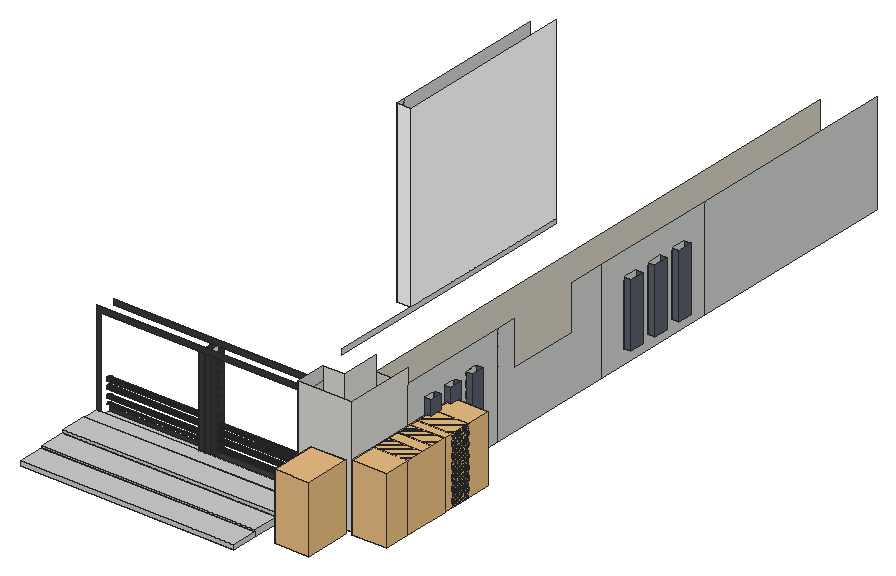
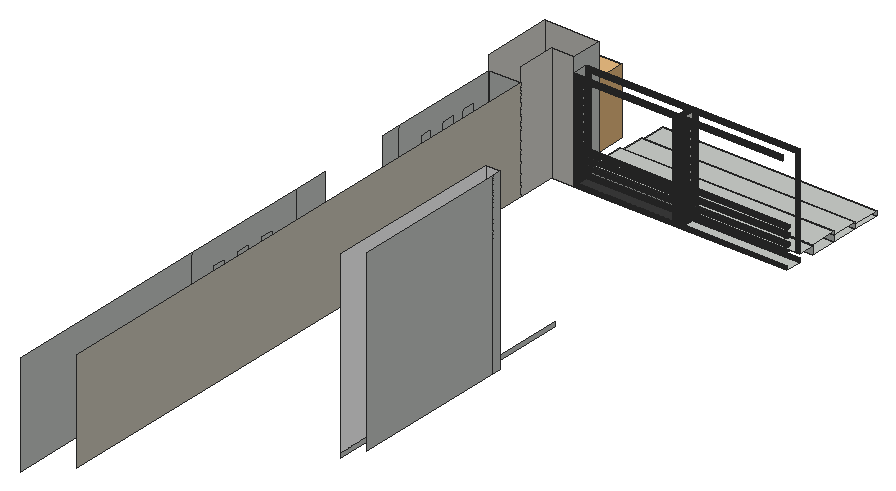
# SketchUp Ruby script. Lengths in inches.
U = 1.inch
M = Sketchup.active_model
def pt(a) = Geom::Point3d.new(a.map { |v| v * U })
def face(e, loops, mat)
  f = e.add_face(loops[0].map { |a| pt(a) })
  loops[1..].each { |l| e.add_face(l.map { |a| pt(a) }).erase! }
  f.material = f.back_material = mat if mat
  f
end
# faces: each face lists its corners as indices into pts; further lists are holes
def faces(e, pts, list, mat = nil) = list.each { |f| face(e, (f[0].is_a?(Array) ? f : [f]).map { |l| l.map { |i| pts[i] } }, mat) }
# xy, xz, yz: faces in a plane at the given z, y or x. An outline is a flat list of corners, or four numbers for a rectangle; further outlines are holes
def ring(l) = l.size == 4 ? [[l[0], l[1]], [l[2], l[1]], [l[2], l[3]], [l[0], l[3]]] : l.each_slice(2).to_a
def flat(e, list, mat, &to3) = list.each { |f| face(e, (f[0].is_a?(Array) ? f : [f]).map { |l| ring(l).map { |u, v| to3.(u, v) } }, mat) }
def xy(e, z, list, mat = nil) = flat(e, list, mat) { |x, y| [x, y, z] }
def xz(e, y, list, mat = nil) = flat(e, list, mat) { |x, z| [x, y, z] }
def yz(e, x, list, mat = nil) = flat(e, list, mat) { |y, z| [x, y, z] }
def lines(e, pts, list) = list.each { |a, b| e.add_line(pt(pts[a]), pt(pts[b])) }
# prism: a flat outline (further loops are holes) pulled along v
def prism(e, loops, v, mat = nil)
  f = face(e, loops, mat); d = Geom::Vector3d.new(v.map { |x| x * U })
  f.pushpull(f.normal.samedirection?(d) ? d.length : -d.length)
end
def box(e, o, s, mat = nil) = prism(e, [[o, [o[0] + s[0], o[1], o[2]], [o[0] + s[0], o[1] + s[1], o[2]], [o[0], o[1] + s[1], o[2]]]], [0, 0, s[2]], mat)
def at(x, y, z, deg = 0) = Geom::Transformation.translation(pt([x, y, z])) * Geom::Transformation.rotation(ORIGIN, Z_AXIS, deg.degrees)
def axes(o, x, y, z) = Geom::Transformation.new([*x, 0, *y, 0, *z, 0, *pt(o).to_a, 1])
def part(name) = M.definitions.add(name)
# library, detail: a bought-in or finely detailed component or shape, given as its bounding box
def library(name, o, s) = part(name).tap { |d| box(d.entities, o, s) }
def detail(e, o, s) = box(e.add_group.entities, o, s)
def put(e, d, t, mat = nil) = e.add_instance(d, t).tap { |i| i.material = mat if mat }
def group(e, t, mat = nil) = e.add_group.tap { |g| g.transformation = t; g.material = mat if mat }.entities
root = M.entities
M.materials.add("[Basic Tile]").color = [203, 206, 202]
M.materials.add("[Color M00]").color = [255, 255, 255]
M.materials.add("[Color M07]").color = [58, 58, 58]
M.materials.add("[Formica Graystone]").color = [209, 204, 189]
M.materials.add("[Formica Laminate Dark]").color = [89, 94, 107]
M.materials.add("[Terrazzo Tile Light]").color = [219, 217, 210]
c1 = library("chau cay",[-24.34,-109.24,0],[56.46,62.58,79.69])
xy(root,0,[[1126.47,137.11,1535.88,187.89],[1126.47,187.89,1535.88,238.67],[1126.47,238.67,1535.88,289.93],[1535.88,289.93,1535.88,350.55,1578.42,350.55,1578.42,424.2,1639.03,424.2,1639.03,289.93],[1126.47,320.24,1535.88,350.55]],"[Basic Tile]")
xy(root,8.3125,[[1322.28,320.24,1333.57,350.55]])
xy(root,8.3125,[[1527,320.24,1535.88,350.55]],"[Basic Tile]")
xy(root,8.3125,[[1344.86,320.24,1527,350.55]],"[Color M07]")
xy(root,8.4375,[[1126.47,137.11,1535.88,187.89]],"[Basic Tile]")
xy(root,11.8125,[[1126.47,187.89,1535.88,238.67]],"[Basic Tile]")
xy(root,15.5,[[1126.47,289.93,1535.88,320.24]],"[Basic Tile]")
xy(root,17.75,[[1126.47,238.67,1535.88,289.93]],"[Basic Tile]")
xy(root,27.29,[[1639.03,943.34,1652.28,971.59],[1639.03,1000.59,1652.28,1028.84],[1639.03,1058.41,1652.28,1086.66]],"[Formica Laminate Dark]")
xy(root,31.8125,[[1639.03,462.79,1652.28,487.66],[1639.03,510.85,1652.28,535.72],[1639.03,562.72,1652.28,587.6]],"[Formica Laminate Dark]")
xz(root,137.11,[[1126.47,0,1535.88,8.4375]],"[Basic Tile]")
xz(root,187.89,[[1126.47,0,1535.88,8.4375],[1126.47,8.4375,1535.88,11.8125]],"[Basic Tile]")
xz(root,238.67,[[1126.47,0,1535.88,11.8125],[1126.47,11.8125,1535.88,17.75]],"[Basic Tile]")
xz(root,289.93,[[1126.47,0,1535.88,15.5],[1126.47,15.5,1535.88,17.75]],"[Basic Tile]")
xz(root,289.93,[[1535.88,0,1639.03,222.4375]],"[Terrazzo Tile Light]")
xz(root,320.24,[[1344.86,8.3125,1527,15.5]],"[Basic Tile]")
xz(root,320.24,[[1126.47,0,1535.88,8.3125],[1322.28,8.3125,1333.57,15.5],[1333.57,8.3125,1344.86,15.5],[1527,8.3125,1535.88,15.5],[1126.47,15.5,1134.85,15.5,1134.85,184.74,1527,184.74,1527,15.5,1535.88,15.5,1535.88,195.17,1126.47,195.17],
  [1322.28,15.5,1333.57,184.74],[1333.57,15.5,1344.86,184.74]],"[Color M07]")
xz(root,350.55,[[1126.47,0,1126.47,8.3125,1333.57,8.3125,1333.57,184.74,1344.86,184.74,1344.86,8.3125,1535.88,8.3125,1535.88,0],[1527,8.3125,1527,184.74,1134.85,184.74,1134.85,195.17,1535.88,195.17,1535.88,8.3125],[1322.28,8.3125,1333.57,184.74]],"[Color M07]")
xz(root,350.55,[[1535.88,0,1578.42,222.4375]],"[Terrazzo Tile Light]")
xz(root,424.2,[[1578.42,0,1639.03,194.8125]],"[Basic Tile]")
xz(root,462.79,[[1639.03,31.8125,1652.28,155.0625]],"[Formica Laminate Dark]")
xz(root,487.66,[[1639.03,31.8125,1652.28,155.0625]],"[Formica Laminate Dark]")
xz(root,510.85,[[1639.03,31.8125,1652.28,155.0625]],"[Formica Laminate Dark]")
xz(root,535.72,[[1639.03,31.8125,1652.28,155.0625]],"[Formica Laminate Dark]")
xz(root,562.72,[[1639.03,31.8125,1652.28,155.0625]],"[Formica Laminate Dark]")
xz(root,587.6,[[1639.03,31.8125,1652.28,155.0625]],"[Formica Laminate Dark]")
xz(root,868.79,[[1262.85,9,1290.28,349.625]],"[Color M00]")
xz(root,943.34,[[1639.03,27.29,1652.28,149.91]],"[Formica Laminate Dark]")
xz(root,971.59,[[1639.03,27.29,1652.28,149.91]],"[Formica Laminate Dark]")
xz(root,1000.59,[[1639.03,27.29,1652.28,149.91]],"[Formica Laminate Dark]")
xz(root,1028.84,[[1639.03,27.29,1652.28,149.91]],"[Formica Laminate Dark]")
xz(root,1058.41,[[1639.03,27.29,1652.28,149.91]],"[Formica Laminate Dark]")
xz(root,1086.66,[[1639.03,27.29,1652.28,149.91]],"[Formica Laminate Dark]")
yz(root,1262.85,[[868.79,9,886.125,349.625],[886.125,9,1187.61,349.625]],"[Basic Tile]")
yz(root,1290.28,[[703.09,0,1215.04,9]],"[Basic Tile]")
yz(root,1290.28,[[868.79,9,1215.04,349.625]],"[Color M00]")
yz(root,1322.28,[[[320.24,8.3125,350.55,184.74],[337.34,16.89,338.33,17.02,339.25,17.4,340.04,18.01,340.64,18.8,341.02,19.72,341.15,20.71,341.02,21.69,340.64,22.61,340.04,23.4,339.25,24.01,338.33,24.39,337.34,24.52,336.35,24.39,335.43,24.01,334.65,23.4,334.04,22.61,333.66,21.69,333.53,20.71,333.66,19.72,334.04,18.8,334.65,18.01,335.43,17.4,336.35,17.02],[337.34,31.39,338.33,31.52,339.25,31.9,340.04,32.51,340.64,33.3,341.02,34.22,341.15,35.21,341.02,36.19,340.64,37.11,340.04,37.9,339.25,38.51,338.33,38.89,337.34,39.02,336.35,38.89,335.43,38.51,334.65,37.9,334.04,37.11,333.66,36.19,333.53,35.21,333.66,34.22,334.04,33.3,334.65,32.51,335.43,31.9,336.35,31.52],[337.34,47.21,338.33,47.34,339.25,47.72,340.04,48.32,340.64,49.11,341.02,50.03,341.15,51.02,341.02,52,340.64,52.92,340.04,53.71,339.25,54.32,338.33,54.7,337.34,54.83,336.35,54.7,335.43,54.32,334.65,53.71,334.04,52.92,333.66,52,333.53,51.02,333.66,50.03,334.04,49.11,334.65,48.32,335.43,47.72,336.35,47.34],[337.34,61.64,338.33,61.77,339.25,62.15,340.04,62.76,340.64,63.55,341.02,64.47,341.15,65.46,341.02,66.44,340.64,67.36,340.04,68.15,339.25,68.76,338.33,69.14,337.34,69.27,336.35,69.14,335.43,68.76,334.65,68.15,334.04,67.36,333.66,66.44,333.53,65.46,333.66,64.47,334.04,63.55,334.65,62.76,335.43,62.15,336.35,61.77],[337.34,76.33,338.33,76.46,339.25,76.84,340.04,77.45,340.64,78.24,341.02,79.16,341.15,80.14,341.02,81.13,340.64,82.05,340.04,82.84,339.25,83.44,338.33,83.83,337.34,83.96,336.35,83.83,335.43,83.44,334.65,82.84,334.04,82.05,333.66,81.13,333.53,80.14,333.66,79.16,334.04,78.24,334.65,77.45,335.43,76.84,336.35,76.46],[337.34,90.83,338.33,90.96,339.25,91.34,340.04,91.95,340.64,92.74,341.02,93.66,341.15,94.64,341.02,95.63,340.64,96.55,340.04,97.34,339.25,97.94,338.33,98.33,337.34,98.46,336.35,98.33,335.43,97.94,334.65,97.34,334.04,96.55,333.66,95.63,333.53,94.64,333.66,93.66,334.04,92.74,334.65,91.95,335.43,91.34,336.35,90.96],[337.34,103.39,338.33,103.52,339.25,103.9,340.04,104.51,340.64,105.3,341.02,106.22,341.15,107.21,341.02,108.19,340.64,109.11,340.04,109.9,339.25,110.51,338.33,110.89,337.34,111.02,336.35,110.89,335.43,110.51,334.65,109.9,334.04,109.11,333.66,108.19,333.53,107.21,333.66,106.22,334.04,105.3,334.65,104.51,335.43,103.9,336.35,103.52],[337.34,117.89,338.33,118.02,339.25,118.4,340.04,119.01,340.64,119.8,341.02,120.72,341.15,121.71,341.02,122.69,340.64,123.61,340.04,124.4,339.25,125.01,338.33,125.39,337.34,125.52,336.35,125.39,335.43,125.01,334.65,124.4,334.04,123.61,333.66,122.69,333.53,121.71,333.66,120.72,334.04,119.8,334.65,119.01,335.43,118.4,336.35,118.02],[337.34,134.02,338.33,134.15,339.25,134.53,340.04,135.13,340.64,135.92,341.02,136.84,341.15,137.83,341.02,138.82,340.64,139.74,340.04,140.53,339.25,141.13,338.33,141.51,337.34,141.64,336.35,141.51,335.43,141.13,334.65,140.53,334.04,139.74,333.66,138.82,333.53,137.83,333.66,136.84,334.04,135.92,334.65,135.13,335.43,134.53,336.35,134.15],[337.34,147.52,338.33,147.65,339.25,148.03,340.04,148.63,340.64,149.42,341.02,150.34,341.15,151.33,341.02,152.32,340.64,153.24,340.04,154.03,339.25,154.63,338.33,155.01,337.34,155.14,336.35,155.01,335.43,154.63,334.65,154.03,334.04,153.24,333.66,152.32,333.53,151.33,333.66,150.34,334.04,149.42,334.65,148.63,335.43,148.03,336.35,147.65],[337.34,161.02,338.33,161.15,339.25,161.53,340.04,162.13,340.64,162.92,341.02,163.84,341.15,164.83,341.02,165.82,340.64,166.74,340.04,167.53,339.25,168.13,338.33,168.51,337.34,168.64,336.35,168.51,335.43,168.13,334.65,167.53,334.04,166.74,333.66,165.82,333.53,164.83,333.66,163.84,334.04,162.92,334.65,162.13,335.43,161.53,336.35,161.15],[337.34,174.52,338.33,174.65,339.25,175.03,340.04,175.63,340.64,176.42,341.02,177.34,341.15,178.33,341.02,179.32,340.64,180.24,340.04,181.03,339.25,181.63,338.33,182.01,337.34,182.14,336.35,182.01,335.43,181.63,334.65,181.03,334.04,180.24,333.66,179.32,333.53,178.33,333.66,177.34,334.04,176.42,334.65,175.63,335.43,175.03,336.35,174.65]]],"[Color M07]")
yz(root,1333.57,[[320.24,8.3125,350.55,184.74]])
yz(root,1344.86,[[[320.24,8.3125,350.55,184.74],[337.76,15.1,336.77,15.23,335.85,15.61,335.06,16.22,334.46,17.01,334.08,17.92,333.95,18.91,334.08,19.9,334.46,20.82,335.06,21.61,335.85,22.21,336.77,22.59,337.76,22.72,338.75,22.59,339.67,22.21,340.46,21.61,341.0625,20.82,341.44,19.9,341.57,18.91,341.44,17.92,341.0625,17.01,340.46,16.22,339.67,15.61,338.75,15.23],[337.76,30.1,336.77,30.23,335.85,30.61,335.06,31.22,334.46,32.01,334.08,32.92,333.95,33.91,334.08,34.9,334.46,35.82,335.06,36.61,335.85,37.21,336.77,37.59,337.76,37.72,338.75,37.59,339.67,37.21,340.46,36.61,341.0625,35.82,341.44,34.9,341.57,33.91,341.44,32.92,341.0625,32.01,340.46,31.22,339.67,30.61,338.75,30.23],[337.76,43.72,336.77,43.85,335.85,44.23,335.06,44.84,334.46,45.63,334.08,46.55,333.95,47.54,334.08,48.52,334.46,49.44,335.06,50.23,335.85,50.84,336.77,51.22,337.76,51.35,338.75,51.22,339.67,50.84,340.46,50.23,341.0625,49.44,341.44,48.52,341.57,47.54,341.44,46.55,341.0625,45.63,340.46,44.84,339.67,44.23,338.75,43.85],[337.76,56.85,336.77,56.98,335.85,57.36,335.06,57.97,334.46,58.76,334.08,59.67,333.95,60.66,334.08,61.65,334.46,62.57,335.06,63.36,335.85,63.96,336.77,64.34,337.76,64.47,338.75,64.34,339.67,63.96,340.46,63.36,341.0625,62.57,341.44,61.65,341.57,60.66,341.44,59.67,341.0625,58.76,340.46,57.97,339.67,57.36,338.75,56.98],[337.76,71.29,336.77,71.42,335.85,71.8,335.06,72.4,334.46,73.19,334.08,74.11,333.95,75.1,334.08,76.09,334.46,77.01,335.06,77.79,335.85,78.4,336.77,78.78,337.76,78.91,338.75,78.78,339.67,78.4,340.46,77.79,341.0625,77.01,341.44,76.09,341.57,75.1,341.44,74.11,341.0625,73.19,340.46,72.4,339.67,71.8,338.75,71.42],[337.76,88.16,336.77,88.29,335.85,88.67,335.06,89.28,334.46,90.07,334.08,90.99,333.95,91.97,334.08,92.96,334.46,93.88,335.06,94.67,335.85,95.28,336.77,95.66,337.76,95.79,338.75,95.66,339.67,95.28,340.46,94.67,341.0625,93.88,341.44,92.96,341.57,91.97,341.44,90.99,341.0625,90.07,340.46,89.28,339.67,88.67,338.75,88.29],[337.76,104.79,336.77,104.92,335.85,105.3,335.06,105.9,334.46,106.69,334.08,107.61,333.95,108.6,334.08,109.59,334.46,110.51,335.06,111.29,335.85,111.9,336.77,112.28,337.76,112.41,338.75,112.28,339.67,111.9,340.46,111.29,341.0625,110.51,341.44,109.59,341.57,108.6,341.44,107.61,341.0625,106.69,340.46,105.9,339.67,105.3,338.75,104.92],[337.76,118.41,336.77,118.54,335.85,118.92,335.06,119.53,334.46,120.32,334.08,121.24,333.95,122.22,334.08,123.21,334.46,124.13,335.06,124.92,335.85,125.53,336.77,125.91,337.76,126.04,338.75,125.91,339.67,125.53,340.46,124.92,341.0625,124.13,341.44,123.21,341.57,122.22,341.44,121.24,341.0625,120.32,340.46,119.53,339.67,118.92,338.75,118.54],[337.76,132.85,336.77,132.98,335.85,133.36,335.06,133.97,334.46,134.76,334.08,135.67,333.95,136.66,334.08,137.65,334.46,138.57,335.06,139.36,335.85,139.96,336.77,140.34,337.76,140.47,338.75,140.34,339.67,139.96,340.46,139.36,341.0625,138.57,341.44,137.65,341.57,136.66,341.44,135.67,341.0625,134.76,340.46,133.97,339.67,133.36,338.75,132.98],[337.76,146.47,336.77,146.6,335.85,146.98,335.06,147.59,334.46,148.38,334.08,149.3,333.95,150.29,334.08,151.27,334.46,152.19,335.06,152.98,335.85,153.59,336.77,153.97,337.76,154.1,338.75,153.97,339.67,153.59,340.46,152.98,341.0625,152.19,341.44,151.27,341.57,150.29,341.44,149.3,341.0625,148.38,340.46,147.59,339.67,146.98,338.75,146.6],[337.76,160.47,336.77,160.6,335.85,160.98,335.06,161.59,334.46,162.38,334.08,163.3,333.95,164.29,334.08,165.27,334.46,166.19,335.06,166.98,335.85,167.59,336.77,167.97,337.76,168.1,338.75,167.97,339.67,167.59,340.46,166.98,341.0625,166.19,341.44,165.27,341.57,164.29,341.44,163.3,341.0625,162.38,340.46,161.59,339.67,160.98,338.75,160.6],[337.76,173.35,336.77,173.48,335.85,173.86,335.06,174.47,334.46,175.26,334.08,176.17,333.95,177.16,334.08,178.15,334.46,179.07,335.06,179.86,335.85,180.46,336.77,180.84,337.76,180.97,338.75,180.84,339.67,180.46,340.46,179.86,341.0625,179.07,341.44,178.15,341.57,177.16,341.44,176.17,341.0625,175.26,340.46,174.47,339.67,173.86,338.75,173.48]]],"[Color M07]")
yz(root,1527,[[337.76,15.1,338.75,15.23,339.67,15.61,340.46,16.22,341.0625,17.01,341.44,17.92,341.57,18.91,341.44,19.9,341.0625,20.82,340.46,21.61,339.67,22.21,338.75,22.59,337.76,22.72,336.77,22.59,335.85,22.21,335.06,21.61,334.46,20.82,334.08,19.9,333.95,18.91,334.08,17.92,334.46,17.01,335.06,16.22,335.85,15.61,336.77,15.23],[337.76,30.1,338.75,30.23,339.67,30.61,340.46,31.22,341.0625,32.01,341.44,32.92,341.57,33.91,341.44,34.9,341.0625,35.82,340.46,36.61,339.67,37.21,338.75,37.59,337.76,37.72,336.77,37.59,335.85,37.21,335.06,36.61,334.46,35.82,334.08,34.9,333.95,33.91,334.08,32.92,334.46,32.01,335.06,31.22,335.85,30.61,336.77,30.23],[337.76,43.72,338.75,43.85,339.67,44.23,340.46,44.84,341.0625,45.63,341.44,46.55,341.57,47.54,341.44,48.52,341.0625,49.44,340.46,50.23,339.67,50.84,338.75,51.22,337.76,51.35,336.77,51.22,335.85,50.84,335.06,50.23,334.46,49.44,334.08,48.52,333.95,47.54,334.08,46.55,334.46,45.63,335.06,44.84,335.85,44.23,336.77,43.85],[337.76,56.85,338.75,56.98,339.67,57.36,340.46,57.97,341.0625,58.76,341.44,59.67,341.57,60.66,341.44,61.65,341.0625,62.57,340.46,63.36,339.67,63.96,338.75,64.34,337.76,64.47,336.77,64.34,335.85,63.96,335.06,63.36,334.46,62.57,334.08,61.65,333.95,60.66,334.08,59.67,334.46,58.76,335.06,57.97,335.85,57.36,336.77,56.98]])
yz(root,1527,[[[320.24,8.3125,350.55,184.74],[337.76,15.1,338.75,15.23,339.67,15.61,340.46,16.22,341.0625,17.01,341.44,17.92,341.57,18.91,341.44,19.9,341.0625,20.82,340.46,21.61,339.67,22.21,338.75,22.59,337.76,22.72,336.77,22.59,335.85,22.21,335.06,21.61,334.46,20.82,334.08,19.9,333.95,18.91,334.08,17.92,334.46,17.01,335.06,16.22,335.85,15.61,336.77,15.23],[337.76,160.47,338.75,160.6,339.67,160.98,340.46,161.59,341.0625,162.38,341.44,163.3,341.57,164.29,341.44,165.27,341.0625,166.19,340.46,166.98,339.67,167.59,338.75,167.97,337.76,168.1,336.77,167.97,335.85,167.59,335.06,166.98,334.46,166.19,334.08,165.27,333.95,164.29,334.08,163.3,334.46,162.38,335.06,161.59,335.85,160.98,336.77,160.6],[337.76,30.1,338.75,30.23,339.67,30.61,340.46,31.22,341.0625,32.01,341.44,32.92,341.57,33.91,341.44,34.9,341.0625,35.82,340.46,36.61,339.67,37.21,338.75,37.59,337.76,37.72,336.77,37.59,335.85,37.21,335.06,36.61,334.46,35.82,334.08,34.9,333.95,33.91,334.08,32.92,334.46,32.01,335.06,31.22,335.85,30.61,336.77,30.23],[337.76,146.47,338.75,146.6,339.67,146.98,340.46,147.59,341.0625,148.38,341.44,149.3,341.57,150.29,341.44,151.27,341.0625,152.19,340.46,152.98,339.67,153.59,338.75,153.97,337.76,154.1,336.77,153.97,335.85,153.59,335.06,152.98,334.46,152.19,334.08,151.27,333.95,150.29,334.08,149.3,334.46,148.38,335.06,147.59,335.85,146.98,336.77,146.6],[337.76,43.72,338.75,43.85,339.67,44.23,340.46,44.84,341.0625,45.63,341.44,46.55,341.57,47.54,341.44,48.52,341.0625,49.44,340.46,50.23,339.67,50.84,338.75,51.22,337.76,51.35,336.77,51.22,335.85,50.84,335.06,50.23,334.46,49.44,334.08,48.52,333.95,47.54,334.08,46.55,334.46,45.63,335.06,44.84,335.85,44.23,336.77,43.85],[337.76,132.85,338.75,132.98,339.67,133.36,340.46,133.97,341.0625,134.76,341.44,135.67,341.57,136.66,341.44,137.65,341.0625,138.57,340.46,139.36,339.67,139.96,338.75,140.34,337.76,140.47,336.77,140.34,335.85,139.96,335.06,139.36,334.46,138.57,334.08,137.65,333.95,136.66,334.08,135.67,334.46,134.76,335.06,133.97,335.85,133.36,336.77,132.98],[337.76,56.85,338.75,56.98,339.67,57.36,340.46,57.97,341.0625,58.76,341.44,59.67,341.57,60.66,341.44,61.65,341.0625,62.57,340.46,63.36,339.67,63.96,338.75,64.34,337.76,64.47,336.77,64.34,335.85,63.96,335.06,63.36,334.46,62.57,334.08,61.65,333.95,60.66,334.08,59.67,334.46,58.76,335.06,57.97,335.85,57.36,336.77,56.98],[337.76,118.41,338.75,118.54,339.67,118.92,340.46,119.53,341.0625,120.32,341.44,121.24,341.57,122.22,341.44,123.21,341.0625,124.13,340.46,124.92,339.67,125.53,338.75,125.91,337.76,126.04,336.77,125.91,335.85,125.53,335.06,124.92,334.46,124.13,334.08,123.21,333.95,122.22,334.08,121.24,334.46,120.32,335.06,119.53,335.85,118.92,336.77,118.54],[337.76,71.29,338.75,71.42,339.67,71.8,340.46,72.4,341.0625,73.19,341.44,74.11,341.57,75.1,341.44,76.09,341.0625,77.01,340.46,77.79,339.67,78.4,338.75,78.78,337.76,78.91,336.77,78.78,335.85,78.4,335.06,77.79,334.46,77.01,334.08,76.09,333.95,75.1,334.08,74.11,334.46,73.19,335.06,72.4,335.85,71.8,336.77,71.42],[337.76,104.79,338.75,104.92,339.67,105.3,340.46,105.9,341.0625,106.69,341.44,107.61,341.57,108.6,341.44,109.59,341.0625,110.51,340.46,111.29,339.67,111.9,338.75,112.28,337.76,112.41,336.77,112.28,335.85,111.9,335.06,111.29,334.46,110.51,334.08,109.59,333.95,108.6,334.08,107.61,334.46,106.69,335.06,105.9,335.85,105.3,336.77,104.92],[337.76,88.16,338.75,88.29,339.67,88.67,340.46,89.28,341.0625,90.07,341.44,90.99,341.57,91.97,341.44,92.96,341.0625,93.88,340.46,94.67,339.67,95.28,338.75,95.66,337.76,95.79,336.77,95.66,335.85,95.28,335.06,94.67,334.46,93.88,334.08,92.96,333.95,91.97,334.08,90.99,334.46,90.07,335.06,89.28,335.85,88.67,336.77,88.29],[337.76,173.35,338.75,173.48,339.67,173.86,340.46,174.47,341.0625,175.26,341.44,176.17,341.57,177.16,341.44,178.15,341.0625,179.07,340.46,179.86,339.67,180.46,338.75,180.84,337.76,180.97,336.77,180.84,335.85,180.46,335.06,179.86,334.46,179.07,334.08,178.15,333.95,177.16,334.08,176.17,334.46,175.26,335.06,174.47,335.85,173.86,336.77,173.48]]],"[Color M07]")
yz(root,1535.88,[[137.11,0,187.89,8.4375],[187.89,0,238.67,11.8125],[238.67,0,289.93,17.75],[289.93,0,320.24,15.5],[320.24,0,350.55,8.3125],
  [320.24,8.3125,350.55,195.17],[289.93,15.5,289.93,222.4375,350.55,222.4375,350.55,195.17,320.24,195.17,320.24,15.5]],"[Basic Tile]")
yz(root,1578.42,[[424.2,0,1486.52,194.8125]],"[Formica Graystone]")
yz(root,1578.42,[[350.55,0,424.2,222.4375]],"[Terrazzo Tile Light]")
yz(root,1639.03,[[[424.2,0,639.97,194.8125],[562.72,31.8125,587.6,155.0625],[510.85,31.8125,535.72,155.0625],[462.79,31.8125,487.66,155.0625]],[639.97,0,888.26,0,888.26,194.8125,818.6,194.8125,818.6,109.0625,679.86,109.0625,679.86,194.8125,639.97,194.8125],[[888.26,0,1135.93,194.8125],[1000.59,27.29,1028.84,149.91],[1058.41,27.29,1086.66,149.91],[943.34,27.29,971.59,149.91]],[1135.93,0,1547.14,194.8125],[943.34,27.29,971.59,149.91],
  [1000.59,27.29,1028.84,149.91],[1058.41,27.29,1086.66,149.91],[462.79,31.8125,487.66,155.0625],[510.85,31.8125,535.72,155.0625],[562.72,31.8125,587.6,155.0625]],"[Basic Tile]")
yz(root,1639.03,[[289.93,0,424.2,222.4375]],"[Terrazzo Tile Light]")
yz(root,1652.28,[[943.34,27.29,971.59,149.91],[1000.59,27.29,1028.84,149.91],[1058.41,27.29,1086.66,149.91],[462.79,31.8125,487.66,155.0625],[510.85,31.8125,535.72,155.0625],
  [562.72,31.8125,587.6,155.0625]],"[Formica Laminate Dark]")
p = [[1527,337.76,15.1],[1527,336.77,15.23],[1344.86,336.77,15.23],[1344.86,337.76,15.1],[1527,338.75,15.23],[1344.86,338.75,15.23],
  [1527,335.85,15.61],[1344.86,335.85,15.61],[1527,339.67,15.61],[1344.86,339.67,15.61],[1527,335.06,16.22],[1344.86,335.06,16.22],
  [1527,340.46,16.22],[1344.86,340.46,16.22],[1527,334.46,17.01],[1344.86,334.46,17.01],[1527,341.0625,17.01],[1344.86,341.0625,17.01],
  [1527,334.08,17.92],[1344.86,334.08,17.92],[1527,341.44,17.92],[1344.86,341.44,17.92],[1527,333.95,18.91],[1344.86,333.95,18.91],
  [1527,341.57,18.91],[1344.86,341.57,18.91],[1527,334.08,19.9],[1344.86,334.08,19.9],[1527,341.44,19.9],[1344.86,341.44,19.9],
  [1527,334.46,20.82],[1344.86,334.46,20.82],[1527,341.0625,20.82],[1344.86,341.0625,20.82],[1527,335.06,21.61],[1344.86,335.06,21.61],
  [1527,340.46,21.61],[1344.86,340.46,21.61],[1527,335.85,22.21],[1344.86,335.85,22.21],[1527,339.67,22.21],[1344.86,339.67,22.21],
  [1527,336.77,22.59],[1344.86,336.77,22.59],[1527,338.75,22.59],[1344.86,338.75,22.59],[1527,337.76,22.72],[1344.86,337.76,22.72],
  [1134.85,335.43,24.01],[1134.85,334.65,23.4],[1322.28,334.65,23.4],[1322.28,335.43,24.01],[1134.85,340.04,23.4],[1134.85,339.25,24.01],
  [1322.28,339.25,24.01],[1322.28,340.04,23.4],[1134.85,336.35,24.39],[1322.28,336.35,24.39],[1134.85,338.33,24.39],[1322.28,338.33,24.39],
  [1134.85,337.34,24.52],[1322.28,337.34,24.52],[1527,337.76,30.1],[1527,336.77,30.23],[1344.86,336.77,30.23],[1344.86,337.76,30.1],
  [1527,338.75,30.23],[1344.86,338.75,30.23],[1527,335.85,30.61],[1344.86,335.85,30.61],[1527,339.67,30.61],[1344.86,339.67,30.61],
  [1527,335.06,31.22],[1344.86,335.06,31.22],[1527,340.46,31.22],[1344.86,340.46,31.22],[1527,334.46,32.01],[1344.86,334.46,32.01],
  [1527,341.0625,32.01],[1344.86,341.0625,32.01],[1134.85,336.35,31.52],[1134.85,337.34,31.39],[1322.28,337.34,31.39],[1322.28,336.35,31.52],
  [1134.85,338.33,31.52],[1322.28,338.33,31.52],[1134.85,335.43,31.9],[1322.28,335.43,31.9],[1134.85,339.25,31.9],[1322.28,339.25,31.9],
  [1134.85,334.65,32.51],[1322.28,334.65,32.51],[1134.85,340.04,32.51],[1322.28,340.04,32.51],[1527,334.08,32.92],[1344.86,334.08,32.92],
  [1527,341.44,32.92],[1344.86,341.44,32.92],[1134.85,334.04,33.3],[1322.28,334.04,33.3],[1134.85,340.64,33.3],[1322.28,340.64,33.3],
  [1527,333.95,33.91],[1344.86,333.95,33.91],[1527,341.57,33.91],[1344.86,341.57,33.91],[1134.85,333.66,34.22],[1322.28,333.66,34.22],
  [1134.85,341.02,34.22],[1322.28,341.02,34.22],[1527,334.08,34.9],[1344.86,334.08,34.9],[1527,341.44,34.9],[1344.86,341.44,34.9],
  [1134.85,333.53,35.21],[1322.28,333.53,35.21],[1134.85,341.15,35.21],[1322.28,341.15,35.21],[1527,334.46,35.82],[1344.86,334.46,35.82],
  [1527,341.0625,35.82],[1344.86,341.0625,35.82],[1134.85,333.66,36.19],[1322.28,333.66,36.19],[1134.85,341.02,36.19],[1322.28,341.02,36.19],
  [1527,335.06,36.61],[1344.86,335.06,36.61],[1527,340.46,36.61],[1344.86,340.46,36.61],[1134.85,334.04,37.11],[1322.28,334.04,37.11],
  [1134.85,340.64,37.11],[1322.28,340.64,37.11],[1527,335.85,37.21],[1344.86,335.85,37.21],[1527,339.67,37.21],[1344.86,339.67,37.21],
  [1134.85,334.65,37.9],[1322.28,334.65,37.9],[1134.85,340.04,37.9],[1322.28,340.04,37.9],[1527,336.77,37.59],[1344.86,336.77,37.59],
  [1527,338.75,37.59],[1344.86,338.75,37.59],[1527,337.76,37.72],[1344.86,337.76,37.72],[1134.85,335.43,38.51],[1322.28,335.43,38.51],
  [1134.85,339.25,38.51],[1322.28,339.25,38.51],[1134.85,336.35,38.89],[1322.28,336.35,38.89],[1134.85,338.33,38.89],[1322.28,338.33,38.89],
  [1134.85,337.34,39.02],[1322.28,337.34,39.02],[1527,337.76,43.72],[1527,336.77,43.85],[1344.86,336.77,43.85],[1344.86,337.76,43.72],
  [1527,338.75,43.85],[1344.86,338.75,43.85],[1527,335.85,44.23],[1344.86,335.85,44.23],[1527,339.67,44.23],[1344.86,339.67,44.23],
  [1527,335.06,44.84],[1344.86,335.06,44.84],[1527,340.46,44.84],[1344.86,340.46,44.84],[1527,334.46,45.63],[1344.86,334.46,45.63],
  [1527,341.0625,45.63],[1344.86,341.0625,45.63],[1527,334.08,46.55],[1344.86,334.08,46.55],[1527,341.44,46.55],[1344.86,341.44,46.55],
  [1527,333.95,47.54],[1344.86,333.95,47.54],[1527,341.57,47.54],[1344.86,341.57,47.54],[1134.85,336.35,47.34],[1134.85,337.34,47.21],
  [1322.28,337.34,47.21],[1322.28,336.35,47.34],[1134.85,338.33,47.34],[1322.28,338.33,47.34],[1134.85,335.43,47.72],[1322.28,335.43,47.72],
  [1134.85,339.25,47.72],[1322.28,339.25,47.72],[1527,334.08,48.52],[1344.86,334.08,48.52],[1527,341.44,48.52],[1344.86,341.44,48.52],
  [1134.85,334.65,48.32],[1322.28,334.65,48.32],[1134.85,340.04,48.32],[1322.28,340.04,48.32],[1134.85,334.04,49.11],[1322.28,334.04,49.11],
  [1134.85,340.64,49.11],[1322.28,340.64,49.11],[1527,334.46,49.44],[1344.86,334.46,49.44],[1527,341.0625,49.44],[1344.86,341.0625,49.44],
  [1134.85,333.66,50.03],[1322.28,333.66,50.03],[1134.85,341.02,50.03],[1322.28,341.02,50.03],[1527,335.06,50.23],[1344.86,335.06,50.23],
  [1527,340.46,50.23],[1344.86,340.46,50.23],[1134.85,333.53,51.02],[1322.28,333.53,51.02],[1134.85,341.15,51.02],[1322.28,341.15,51.02],
  [1527,335.85,50.84],[1344.86,335.85,50.84],[1527,339.67,50.84],[1344.86,339.67,50.84],[1527,336.77,51.22],[1344.86,336.77,51.22],
  [1527,338.75,51.22],[1344.86,338.75,51.22],[1134.85,333.66,52],[1322.28,333.66,52],[1134.85,341.02,52],[1322.28,341.02,52],
  [1527,337.76,51.35],[1344.86,337.76,51.35],[1134.85,334.04,52.92],[1322.28,334.04,52.92],[1134.85,340.64,52.92],[1322.28,340.64,52.92],
  [1134.85,334.65,53.71],[1322.28,334.65,53.71],[1134.85,340.04,53.71],[1322.28,340.04,53.71],[1134.85,335.43,54.32],[1322.28,335.43,54.32],
  [1134.85,339.25,54.32],[1322.28,339.25,54.32],[1134.85,336.35,54.7],[1322.28,336.35,54.7],[1134.85,338.33,54.7],[1322.28,338.33,54.7],
  [1134.85,337.34,54.83],[1322.28,337.34,54.83],[1527,337.76,56.85],[1527,336.77,56.98],[1344.86,336.77,56.98],[1344.86,337.76,56.85],
  [1527,338.75,56.98],[1344.86,338.75,56.98],[1527,335.85,57.36],[1344.86,335.85,57.36],[1527,339.67,57.36],[1344.86,339.67,57.36],
  [1527,335.06,57.97],[1344.86,335.06,57.97],[1527,340.46,57.97],[1344.86,340.46,57.97],[1527,334.46,58.76],[1344.86,334.46,58.76],
  [1527,341.0625,58.76],[1344.86,341.0625,58.76],[1527,334.08,59.67],[1344.86,334.08,59.67],[1527,341.44,59.67],[1344.86,341.44,59.67],
  [1527,333.95,60.66],[1344.86,333.95,60.66],[1527,341.57,60.66],[1344.86,341.57,60.66],[1527,334.08,61.65],[1344.86,334.08,61.65],
  [1527,341.44,61.65],[1344.86,341.44,61.65],[1527,334.46,62.57],[1344.86,334.46,62.57],[1134.85,336.35,61.77],[1134.85,337.34,61.64],
  [1322.28,337.34,61.64],[1322.28,336.35,61.77],[1134.85,338.33,61.77],[1322.28,338.33,61.77],[1527,341.0625,62.57],[1344.86,341.0625,62.57],
  [1134.85,335.43,62.15],[1322.28,335.43,62.15],[1134.85,339.25,62.15],[1322.28,339.25,62.15],[1134.85,334.65,62.76],[1322.28,334.65,62.76],
  [1134.85,340.04,62.76],[1322.28,340.04,62.76],[1527,335.06,63.36],[1344.86,335.06,63.36],[1527,340.46,63.36],[1344.86,340.46,63.36],
  [1134.85,334.04,63.55],[1322.28,334.04,63.55],[1134.85,340.64,63.55],[1322.28,340.64,63.55],[1527,335.85,63.96],[1344.86,335.85,63.96],
  [1527,339.67,63.96],[1344.86,339.67,63.96],[1134.85,333.66,64.47],[1322.28,333.66,64.47],[1134.85,341.02,64.47],[1322.28,341.02,64.47],
  [1527,336.77,64.34],[1344.86,336.77,64.34],[1527,338.75,64.34],[1344.86,338.75,64.34],[1527,337.76,64.47],[1344.86,337.76,64.47],
  [1134.85,333.53,65.46],[1322.28,333.53,65.46],[1134.85,341.15,65.46],[1322.28,341.15,65.46],[1134.85,333.66,66.44],[1322.28,333.66,66.44],
  [1134.85,341.02,66.44],[1322.28,341.02,66.44],[1134.85,334.04,67.36],[1322.28,334.04,67.36],[1134.85,340.64,67.36],[1322.28,340.64,67.36],
  [1134.85,334.65,68.15],[1322.28,334.65,68.15],[1134.85,340.04,68.15],[1322.28,340.04,68.15],[1134.85,335.43,68.76],[1322.28,335.43,68.76],
  [1134.85,339.25,68.76],[1322.28,339.25,68.76]]
faces(root,p,[[0,1,2,3],[4,0,3,5],[1,6,7,2],[8,4,5,9],[6,10,11,7],[12,8,9,13],[10,14,15,11],[16,12,13,17],
  [14,18,19,15],[20,16,17,21],[18,22,23,19],[24,20,21,25],[22,26,27,23],[28,24,25,29],[26,30,31,27],[32,28,29,33],
  [30,34,35,31],[36,32,33,37],[34,38,39,35],[40,36,37,41],[38,42,43,39],[44,40,41,45],[42,46,47,43],[46,44,45,47],
  [48,49,50,51],[52,53,54,55],[56,48,51,57],[53,58,59,54],[60,56,57,61],[58,60,61,59],[62,63,64,65],[66,62,65,67],
  [63,68,69,64],[70,66,67,71],[68,72,73,69],[74,70,71,75],[72,76,77,73],[78,74,75,79],[80,81,82,83],[81,84,85,82],
  [86,80,83,87],[84,88,89,85],[90,86,87,91],[88,92,93,89],[76,94,95,77],[96,78,79,97],[98,90,91,99],[92,100,101,93],
  [94,102,103,95],[104,96,97,105],[106,98,99,107],[100,108,109,101],[102,110,111,103],[112,104,105,113],[114,106,107,115],[108,116,117,109],
  [110,118,119,111],[120,112,113,121],[122,114,115,123],[116,124,125,117],[118,126,127,119],[128,120,121,129],[130,122,123,131],[124,132,133,125],
  [126,134,135,127],[136,128,129,137],[138,130,131,139],[132,140,141,133],[134,142,143,135],[144,136,137,145],[142,146,147,143],[146,144,145,147],
  [148,138,139,149],[140,150,151,141],[152,148,149,153],[150,154,155,151],[156,152,153,157],[154,156,157,155],[158,159,160,161],[162,158,161,163],
  [159,164,165,160],[166,162,163,167],[164,168,169,165],[170,166,167,171],[168,172,173,169],[174,170,171,175],[172,176,177,173],[178,174,175,179],
  [176,180,181,177],[182,178,179,183],[184,185,186,187],[185,188,189,186],[190,184,187,191],[188,192,193,189],[180,194,195,181],[196,182,183,197],
  [198,190,191,199],[192,200,201,193],[202,198,199,203],[200,204,205,201],[194,206,207,195],[208,196,197,209],[210,202,203,211],[204,212,213,205],
  [206,214,215,207],[216,208,209,217],[218,210,211,219],[212,220,221,213],[214,222,223,215],[224,216,217,225],[222,226,227,223],[228,224,225,229],
  [230,218,219,231],[220,232,233,221],[226,234,235,227],[234,228,229,235],[236,230,231,237],[232,238,239,233],[240,236,237,241],[238,242,243,239],
  [244,240,241,245],[242,246,247,243],[248,244,245,249],[246,250,251,247],[252,248,249,253],[250,252,253,251],[254,255,256,257],[258,254,257,259],
  [255,260,261,256],[262,258,259,263],[260,264,265,261],[266,262,263,267],[264,268,269,265],[270,266,267,271],[268,272,273,269],[274,270,271,275],
  [272,276,277,273],[278,274,275,279],[276,280,281,277],[282,278,279,283],[280,284,285,281],[286,287,288,289],[287,290,291,288],[292,282,283,293],
  [294,286,289,295],[290,296,297,291],[298,294,295,299],[296,300,301,297],[284,302,303,285],[304,292,293,305],[306,298,299,307],[300,308,309,301],
  [302,310,311,303],[312,304,305,313],[314,306,307,315],[308,316,317,309],[310,318,319,311],[320,312,313,321],[318,322,323,319],[322,320,321,323],
  [324,314,315,325],[316,326,327,317],[328,324,325,329],[326,330,331,327],[332,328,329,333],[330,334,335,331],[336,332,333,337],[334,338,339,335],
  [340,336,337,341],[338,342,343,339]],"[Color M07]")
put(root,c1,axes([1599.82,343.48,0],[1.17,0,0],[0,1.4,0],[0,0,1.6]))
put(root,c1,axes([1673.59,436.24,0],[1.17,0,0],[0,1.4,0],[0,0,1.6]))
put(root,c1,axes([1673.59,487.99,0],[1.17,0,0],[0,1.4,0],[0,0,1.6]))
put(root,c1,axes([1673.59,545.55,0],[1.17,0,0],[0,1.4,0],[0,0,1.6]))
put(root,c1,axes([1673.59,592.36,0],[1.17,0,0],[0,1.4,0],[0,0,1.6]))
